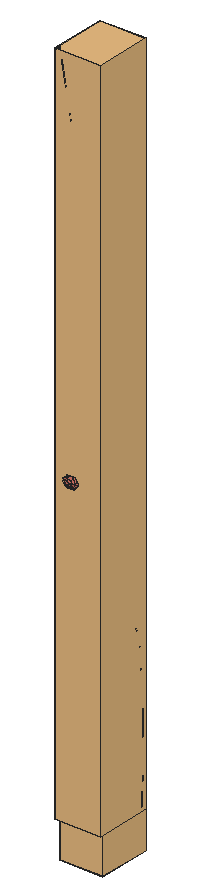
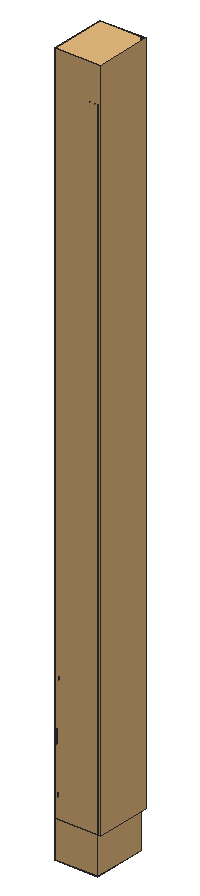
# SketchUp Ruby script. Lengths in inches.
U = 1.inch
M = Sketchup.active_model
def pt(a) = Geom::Point3d.new(a.map { |v| v * U })
def face(e, loops, mat)
  f = e.add_face(loops[0].map { |a| pt(a) })
  loops[1..].each { |l| e.add_face(l.map { |a| pt(a) }).erase! }
  f.material = f.back_material = mat if mat
  f
end
# faces: each face lists its corners as indices into pts; further lists are holes
def faces(e, pts, list, mat = nil) = list.each { |f| face(e, (f[0].is_a?(Array) ? f : [f]).map { |l| l.map { |i| pts[i] } }, mat) }
# xy, xz, yz: faces in a plane at the given z, y or x. An outline is a flat list of corners, or four numbers for a rectangle; further outlines are holes
def ring(l) = l.size == 4 ? [[l[0], l[1]], [l[2], l[1]], [l[2], l[3]], [l[0], l[3]]] : l.each_slice(2).to_a
def flat(e, list, mat, &to3) = list.each { |f| face(e, (f[0].is_a?(Array) ? f : [f]).map { |l| ring(l).map { |u, v| to3.(u, v) } }, mat) }
def xy(e, z, list, mat = nil) = flat(e, list, mat) { |x, y| [x, y, z] }
def xz(e, y, list, mat = nil) = flat(e, list, mat) { |x, z| [x, y, z] }
def yz(e, x, list, mat = nil) = flat(e, list, mat) { |y, z| [x, y, z] }
def lines(e, pts, list) = list.each { |a, b| e.add_line(pt(pts[a]), pt(pts[b])) }
# prism: a flat outline (further loops are holes) pulled along v
def prism(e, loops, v, mat = nil)
  f = face(e, loops, mat); d = Geom::Vector3d.new(v.map { |x| x * U })
  f.pushpull(f.normal.samedirection?(d) ? d.length : -d.length)
end
def box(e, o, s, mat = nil) = prism(e, [[o, [o[0] + s[0], o[1], o[2]], [o[0] + s[0], o[1] + s[1], o[2]], [o[0], o[1] + s[1], o[2]]]], [0, 0, s[2]], mat)
def at(x, y, z, deg = 0) = Geom::Transformation.translation(pt([x, y, z])) * Geom::Transformation.rotation(ORIGIN, Z_AXIS, deg.degrees)
def axes(o, x, y, z) = Geom::Transformation.new([*x, 0, *y, 0, *z, 0, *pt(o).to_a, 1])
def part(name) = M.definitions.add(name)
# library, detail: a bought-in or finely detailed component or shape, given as its bounding box
def library(name, o, s) = part(name).tap { |d| box(d.entities, o, s) }
def detail(e, o, s) = box(e.add_group.entities, o, s)
def put(e, d, t, mat = nil) = e.add_instance(d, t).tap { |i| i.material = mat if mat }
def group(e, t, mat = nil) = e.add_group.tap { |g| g.transformation = t; g.material = mat if mat }.entities
root = M.entities
M.materials.add("green").color = [174, 139, 102]
M.materials.add("vio").color = [206, 114, 100]
c1 = part("3DGeom~209_Defintion")
p = [[-82.63,99.78,-479.67],[16.24,-187.65,-448.99],[-197.0625,-62.73,-454.35],[148.38,0,-478.24],[-291.5,172.82,-352.58],[-2.625,262.29,-394.02],
  [-245.31,266.64,-303.125],[-291.5,172.82,-352.58],[-245.31,266.64,-303.125],[225.19,-262.29,-323.34],[339.63,-99.78,-348.66],[240.76,187.65,-379.34],
  [-120.25,-325.02,-299.44],[-315.27,-181.7,-324.83],[-120.25,-325.02,-299.44],[-357.57,78.99,-337.96],[-315.27,-181.7,-324.83],[-291.5,172.82,-352.58],
  [-357.57,78.99,-337.96],[106.99,-381.25,-193.82],[-120.25,-325.02,-299.44],[106.99,-381.25,-193.82],[21.51,381.25,-220.34],[-231.37,335.33,-202.85],
  [-2.625,262.29,-394.02],[-245.31,266.64,-303.125],[-231.37,335.33,-202.85],[21.51,381.25,-220.34],[-2.625,262.29,-394.02],[419.63,62.73,-263.01],
  [268.63,325.02,-178.79],[419.63,62.73,-263.01],[240.76,187.65,-379.34],[21.51,381.25,-220.34],[268.63,325.02,-178.79],[-291.5,172.82,-352.58],
  [-357.57,78.99,-337.96],[-422.26,199.55,-131.01],[-245.31,266.64,-303.125],[339.63,-99.78,-348.66],[373.81,-266.64,-111.04],[225.19,-262.29,-323.34],
  [339.63,-99.78,-348.66],[439.875,-172.82,-125.66],[373.81,-266.64,-111.04],[419.63,62.73,-263.01],[339.63,-99.78,-348.66],[-357.57,78.99,-337.96],
  [-315.27,-181.7,-324.83],[-425.81,10.31,-263.18],[-425.81,10.31,-263.18],[-315.27,-181.7,-324.83],[-224.52,-375.3,-69.66],[-405.57,-225.25,-125.83],
  [-315.27,-181.7,-324.83],[-120.25,-325.02,-299.44],[-315.27,-181.7,-324.83],[-405.57,-225.25,-125.83],[225.19,-262.29,-323.34],[305.5625,-335.33,-36.26],
  [106.99,-381.25,-193.82],[225.19,-262.29,-323.34],[373.81,-266.64,-111.04],[-231.37,335.33,-202.85],[16.69,-424.8,5.18],[-477.94,-14.83,-148.29],
  [419.63,62.73,-263.01],[486.07,-78.99,-76.21],[443.77,181.7,-89.33],[419.63,62.73,-263.01],[268.63,325.02,-178.79],[419.63,62.73,-263.01],
  [-16.69,424.8,-5.18],[268.63,325.02,-178.79],[-253.43,360.47,-78.63],[-231.37,335.33,-202.85],[-253.43,360.47,-78.63],[-253.43,360.47,-78.63],
  [253.43,-360.47,78.63],[224.52,375.3,69.66],[268.63,325.02,-178.79],[224.52,375.3,69.66],[268.63,325.02,-178.79],[-443.77,-181.7,89.33],
  [-500,10.31,-24.0625],[-486.07,78.99,76.21],[-439.875,172.82,125.66],[-373.81,266.64,111.04],[-305.5625,335.33,36.26],[-224.52,-375.3,-69.66],
  [-268.63,-325.02,178.79],[373.81,-266.64,-111.04],[422.26,-199.55,131.01],[305.5625,-335.33,-36.26],[373.81,-266.64,-111.04],[500,-10.31,24.0625],
  [405.57,225.25,125.83],[224.52,375.3,69.66],[-305.5625,335.33,36.26],[-253.43,360.47,-78.63],[-21.51,-381.25,220.34],[-21.51,-381.25,220.34],
  [-268.63,-325.02,178.79],[253.43,-360.47,78.63],[305.5625,-335.33,-36.26],[-419.63,-62.73,263.01],[-305.5625,335.33,36.26],[-106.99,381.25,193.82],
  [231.37,-335.33,202.85],[-21.51,-381.25,220.34],[477.94,14.83,148.29],[-373.81,266.64,111.04],[-305.5625,335.33,36.26],[120.25,325.02,299.44],
  [405.57,225.25,125.83],[-339.63,99.78,348.66],[231.37,-335.33,202.85],[253.43,-360.47,78.63],[-240.76,-187.65,379.34],[-240.76,-187.65,379.34],
  [-225.19,262.29,323.34],[-373.81,266.64,111.04],[-225.19,262.29,323.34],[-225.19,262.29,323.34],[315.27,181.7,324.83],[315.27,181.7,324.83],
  [405.57,225.25,125.83],[245.31,-266.64,303.125],[231.37,-335.33,202.85],[291.5,-172.82,352.58],[245.31,-266.64,303.125],[357.57,-78.99,337.96],
  [291.5,-172.82,352.58],[425.81,-10.31,263.18],[357.57,-78.99,337.96],[315.27,181.7,324.83],[-268.63,-325.02,178.79],[-21.51,-381.25,220.34],
  [2.625,-262.29,394.02],[-268.63,-325.02,178.79],[-240.76,-187.65,379.34],[-225.19,262.29,323.34],[120.25,325.02,299.44],[-106.99,381.25,193.82],
  [-21.51,-381.25,220.34],[245.31,-266.64,303.125],[-21.51,-381.25,220.34],[245.31,-266.64,303.125],[2.625,-262.29,394.02],[-419.63,-62.73,263.01],
  [-148.38,0,478.24],[-419.63,-62.73,263.01],[-339.63,99.78,348.66],[197.0625,62.74,454.35],[357.57,-78.99,337.96],[425.81,-10.31,263.18],
  [425.81,-10.31,263.18],[315.27,181.7,324.83],[-16.24,187.65,448.99],[315.27,181.7,324.83],[120.25,325.02,299.44],[-225.19,262.29,323.34],
  [120.25,325.02,299.44],[245.31,-266.64,303.125],[291.5,-172.82,352.58],[-339.63,99.78,348.66],[-225.19,262.29,323.34],[315.27,181.7,324.83],
  [82.63,-99.77,479.67],[-339.63,99.78,348.66]]
faces(c1.entities,p,[[0,1,2],[0,3,1],[4,0,2],[5,3,0],[6,0,7],[8,5,0],[3,9,1],[3,10,9],
  [11,10,3],[5,11,3],[2,12,13],[2,1,14],[15,2,16],[17,2,18],[1,19,20],[1,9,21],
  [22,11,5],[23,24,25],[26,27,28],[11,29,10],[30,31,32],[33,34,11],[35,36,37],[38,35,37],
  [39,40,41],[42,43,44],[45,43,46],[47,48,49],[36,50,37],[51,52,53],[54,55,52],[50,56,57],
  [58,59,60],[61,62,59],[63,38,37],[55,64,52],[55,60,64],[50,57,65],[50,65,37],[66,67,43],
  [68,67,69],[70,68,71],[72,73,27],[74,27,75],[76,72,27],[77,63,37],[60,78,64],[60,59,78],
  [79,68,80],[72,81,82],[65,57,83],[65,83,84],[65,84,37],[84,85,37],[85,86,37],[86,87,37],
  [88,77,37],[87,88,37],[57,89,90],[57,90,83],[91,43,92],[43,67,92],[93,94,92],[68,95,67],
  [96,95,68],[97,96,68],[98,72,99],[67,95,92],[52,64,100],[52,101,102],[103,104,92],[84,83,105],
  [84,105,85],[106,107,72],[107,81,72],[64,108,109],[64,78,108],[95,110,92],[96,110,95],[111,107,112],
  [113,114,81],[107,113,81],[85,105,115],[85,115,86],[116,117,92],[83,90,118],[83,119,105],[86,120,87],
  [121,122,107],[86,115,123],[124,110,96],[113,125,126],[127,128,92],[129,130,92],[131,132,92],[133,134,92],
  [110,133,92],[135,133,110],[136,137,138],[139,138,140],[141,142,143],[144,108,145],[146,147,148],[149,140,150],
  [151,150,152],[153,154,155],[153,156,157],[158,159,160],[161,158,162],[138,163,164],[165,158,166],[158,153,167],
  [168,164,154],[168,154,153],[169,150,158],[138,164,168],[140,138,168],[140,168,150],[150,153,158],[150,168,153]],"vio")
c2 = part("3DGeom~162_Defintion")
p = [[24.5,499.67,-28.18],[34.6875,499.96,-22.61],[27.51,499.8125,-29.5],[24.5,499.67,-28.18],[27.51,499.8125,-29.5],[25.94,499.74,-29.06],
  [27.51,499.8125,-29.5],[34.6875,499.96,-22.61],[30.68,499.93,-29.16],[27.51,499.8125,-29.5],[30.68,499.93,-29.16],[29.11,499.875,-29.54],
  [30.68,499.93,-29.16],[34.6875,499.96,-22.61],[33.33,499.99,-27.23],[30.68,499.93,-29.16],[33.33,499.99,-27.23],[32.11,499.97,-28.39],
  [22.58,499.54,-25.53],[34.6875,499.96,-22.61],[24.5,499.67,-28.18],[22.58,499.54,-25.53],[24.5,499.67,-28.18],[23.34,499.6,-26.96],
  [33.33,499.99,-27.23],[34.6875,499.96,-22.61],[34.66,499.99,-24.22],[33.33,499.99,-27.23],[34.66,499.99,-24.22],[34.21,500,-25.79],
  [22.24,499.47,-22.35],[34.6875,499.96,-22.61],[22.58,499.54,-25.53],[22.24,499.47,-22.35],[22.58,499.54,-25.53],[22.2,499.5,-23.96],
  [23.56,499.46,-19.35],[34.6875,499.96,-22.61],[22.24,499.47,-22.35],[26.22,499.53,-17.41],[34.6875,499.96,-22.61],[23.56,499.46,-19.35],
  [34.32,499.91,-21.05],[34.6875,499.96,-22.61],[26.22,499.53,-17.41],[23.56,499.46,-19.35],[22.24,499.47,-22.35],[22.6875,499.46,-20.79],
  [34.32,499.91,-21.05],[26.22,499.53,-17.41],[27.78,499.58,-17.04],[30.95,499.72,-17.52],[34.32,499.91,-21.05],[27.78,499.58,-17.04],
  [32.39,499.79,-18.39],[34.32,499.91,-21.05],[30.95,499.72,-17.52],[32.39,499.79,-18.39],[33.55,499.86,-19.61],[34.32,499.91,-21.05],
  [26.22,499.53,-17.41],[23.56,499.46,-19.35],[24.78,499.49,-18.1875],[30.95,499.72,-17.52],[27.78,499.58,-17.04],[29.39,499.65,-17.07],
  [-36.91,-499.89,26.6875],[-36.31,-499.93,26.63],[-35.71,-499.97,26.73],[-36.91,-499.89,26.6875],[-35.71,-499.97,26.73],[-34.01,-499.94,29.09],
  [-35.71,-499.97,26.73],[-35.15,-499.99,26.99],[-34.65,-500,27.39],[-35.71,-499.97,26.73],[-34.65,-500,27.39],[-34.01,-499.94,29.09],
  [-38,-499.78,27.26],[-37.49,-499.83,26.9],[-36.91,-499.89,26.6875],[-38,-499.78,27.26],[-36.91,-499.89,26.6875],[-34.01,-499.94,29.09],
  [-38.66,-499.67,28.32],[-38,-499.78,27.26],[-34.01,-499.94,29.09],[-38.66,-499.67,28.32],[-38.41,-499.72,27.75],[-38,-499.78,27.26],
  [-34.65,-500,27.39],[-34.29,-499.99,27.91],[-34.07,-499.97,28.49],[-34.65,-500,27.39],[-34.07,-499.97,28.49],[-34.01,-499.94,29.09],
  [-38.69,-499.59,29.52],[-38.66,-499.67,28.32],[-34.01,-499.94,29.09],[-38.69,-499.59,29.52],[-38.75,-499.625,28.91],[-38.66,-499.67,28.32],
  [-38.11,-499.57,30.62],[-38.69,-499.59,29.52],[-34.01,-499.94,29.09],[-37.06,-499.6,31.27],[-38.11,-499.57,30.62],[-34.01,-499.94,29.09],
  [-34.11,-499.9,29.69],[-37.06,-499.6,31.27],[-34.01,-499.94,29.09],[-38.11,-499.57,30.62],[-38.48,-499.57,30.1],[-38.69,-499.59,29.52],
  [-34.11,-499.9,29.69],[-36.46,-499.64,31.375],[-37.06,-499.6,31.27],[-35.28,-499.73,31.11],[-36.46,-499.64,31.375],[-34.11,-499.9,29.69],
  [-34.11,-499.9,29.69],[-34.76,-499.79,30.74],[-35.28,-499.73,31.11],[-34.11,-499.9,29.69],[-34.36,-499.85,30.25],[-34.76,-499.79,30.74],
  [-37.06,-499.6,31.27],[-37.62,-499.58,31.02],[-38.11,-499.57,30.62],[-35.28,-499.73,31.11],[-35.86,-499.68,31.32],[-36.46,-499.64,31.375]]
faces(c2.entities,p,[[0,1,2],[3,4,5],[6,7,8],[9,10,11],[12,13,14],[15,16,17],[18,19,20],[21,22,23],
  [24,25,26],[27,28,29],[30,31,32],[33,34,35],[36,37,38],[39,40,41],[42,43,44],[45,46,47],
  [48,49,50],[51,52,53],[54,55,56],[57,58,59],[60,61,62],[63,64,65],[66,67,68],[69,70,71],
  [72,73,74],[75,76,77],[78,79,80],[81,82,83],[84,85,86],[87,88,89],[90,91,92],[93,94,95],
  [96,97,98],[99,100,101],[102,103,104],[105,106,107],[108,109,110],[111,112,113],[114,115,116],[117,118,119],
  [120,121,122],[123,124,125],[126,127,128],[129,130,131]],"green")
c3 = library("3DGeom~76_Defintion",[-357.42,-500,-94.02],[714.84,1000,188.04])
c4 = part("3DGeom~77_Defintion")
p = [[339.625,495.99,-59.28],[344.32,486.75,-93.94],[336.28,491.02,-94.02],[339.625,495.99,-59.28],[336.28,491.02,-94.02],[329.77,495.38,-89.43],
  [339.625,495.99,-59.28],[351.73,483.72,-89.22],[344.32,486.75,-93.94],[339.625,495.99,-59.28],[329.77,495.38,-89.43],[326.53,498.67,-81.4],
  [339.625,495.99,-59.28],[356.52,482.74,-81.125],[351.73,483.72,-89.22],[339.625,495.99,-59.28],[326.53,498.67,-81.4],[327.42,500,-72.09],
  [339.625,495.99,-59.28],[357.42,484.07,-71.82],[356.52,482.74,-81.125],[339.625,495.99,-59.28],[327.42,500,-72.09],[332.22,499.02,-64],
  [339.625,495.99,-59.28],[354.18,487.36,-63.79],[357.42,484.07,-71.82],[339.625,495.99,-59.28],[347.66,491.72,-59.2],[354.18,487.36,-63.79],
  [-333.46,-489.29,27.51],[-350.37,-484.43,31.63],[-342.13,-486.03,27.33],[-323.61,-497.07,39.94],[-347.57,-495.14,60.61],[-333.46,-489.29,27.51],
  [-323.61,-497.07,39.94],[-333.46,-489.29,27.51],[-326.68,-493.33,32.125],[-333.46,-489.29,27.51],[-347.57,-495.14,60.61],[-350.37,-484.43,31.63],
  [-350.37,-484.43,31.63],[-347.57,-495.14,60.61],[-357.42,-487.36,48.18],[-350.37,-484.43,31.63],[-357.42,-487.36,48.18],[-355.96,-484.92,39.27],
  [-330.67,-500,56.48],[-347.57,-495.14,60.61],[-323.61,-497.07,39.94],[-330.67,-500,56.48],[-323.61,-497.07,39.94],[-325.07,-499.51,48.85],
  [-347.57,-495.14,60.61],[-354.35,-491.1,55.99],[-357.42,-487.36,48.18],[-347.57,-495.14,60.61],[-330.67,-500,56.48],[-338.9,-498.4,60.79]]
faces(c4.entities,p,[[0,1,2],[3,4,5],[6,7,8],[9,10,11],[12,13,14],[15,16,17],[18,19,20],[21,22,23],
  [24,25,26],[27,28,29],[30,31,32],[33,34,35],[36,37,38],[39,40,41],[42,43,44],[45,46,47],
  [48,49,50],[51,52,53],[54,55,56],[57,58,59]],"green")
c5 = library("3DGeom~161_Defintion",[-40.83,-526.88,-33.06],[81.66,1000,66.12])
c6 = library("3DGeom~158_Defintion",[-40.84,-526.87,-33.0625],[81.68,1000,66.125])
c7 = part("3DGeom~155_Defintion")
p = [[38.32,377.89,-31.94],[39.08,336.41,-30.625],[37.92,336.42,-31.72],[39.51,377.89,-30.8125],[36.28,473.1,-31.04],[39,423.46,-30.56],
  [37.77,423.45,-31.72],[36.57,299.05,-31.05],[35.37,265.71,-28.9],[34.28,265.75,-29.93],[37.7,299.02,-29.98],[37.54,473.12,-29.85],
  [30.51,238.44,-28.47],[26.13,217.53,-25.5625],[25.09,217.6875,-26.58],[31.58,238.34,-27.4375],[18.69,201.11,-24.24],[13.09,186.1875,-20.43],
  [12.09,186.36,-21.43],[19.71,200.92,-23.23],[17.34,-63.12,-14.97],[21.97,-83.66,-18.45],[21.09,-83.65,-19.17],[20.41,-107.24,-19.11],
  [17.68,-132.65,-15.82],[16.86,-132.61,-16.5],[21.25,-107.27,-18.41],[18.22,-63.09,-14.24],[5.95,170.98,-18.125],[1.85,152.3,-13.32],
  [0.82,152.32,-14.25],[6.97,170.87,-17.16],[11.42,-160.05,-12.18],[5.8,-189.86,-6.34],[5.02,-189.82,-6.98],[12.22,-160.09,-11.52],
  [-4.11,129.18,-8.57],[-8.33,104.16,-0.18],[-9.33,104.1,-1.06],[-3.09,129.2,-7.66],[0.27,-33.7,2.54],[10.55,-46.99,-6.22],
  [9.67,-47.04,-6.98],[1.16,-33.64,3.32],[-1.41,-222.19,-1.7],[-6.22,-257.42,3.45],[-6.96,-257.4,2.85],[-0.65,-222.22,-1.08],
  [-11.84,-295.59,6.88],[-16.11,-336.49,11.55],[-16.77,-336.48,11.01],[-11.14,-295.61,7.45],[-14.18,78.26,6.96],[-17,52.91,15.01],
  [-17.97,52.84,14.16],[-13.19,78.33,7.82],[-16.02,-7.84,18.13],[-7.97,-21.15,12.31],[-8.87,-21.22,11.51],[-15.1,-7.78,18.9375],
  [-21.76,-380.05,15.23],[-26.21,-426.32,20.02],[-26.8,-426.3,19.54],[-21.13,-380.0625,15.74],[-20.06,29.08,19.25],[-18.85,8.375,21.75],
  [-19.78,8.33,20.94],[-19.1,29.15,20.08],[-31.89,-475.25,23.94],[-36.52,-526.88,28.86],[-37.04,-526.87,28.4375],[-31.34,-475.26,24.4]]
faces(c7.entities,p,[[0,1,2],[0,3,1],[4,5,6],[7,8,9],[7,10,8],[4,11,5],[12,13,14],[12,15,13],
  [16,17,18],[16,19,17],[20,21,22],[23,24,25],[23,26,24],[20,27,21],[28,29,30],[28,31,29],
  [32,33,34],[32,35,33],[36,37,38],[36,39,37],[40,41,42],[40,43,41],[44,45,46],[44,47,45],
  [48,49,50],[48,51,49],[52,53,54],[52,55,53],[56,57,58],[56,59,57],[60,61,62],[60,63,61],
  [64,65,66],[64,67,65],[68,69,70],[68,71,69]],"green")
c8 = part("3DGeom~159_Defintion")
p = [[36.92,377.89,-32.7],[37.92,336.42,-31.72],[36.56,336.4375,-32.45],[38.32,377.89,-31.94],[34.8,473.07,-31.83],[37.77,423.44,-31.72],
  [36.34,423.43,-32.49],[35.25,299.08,-31.77],[34.28,265.75,-29.93],[32.99,265.81,-30.625],[36.57,299.05,-31.05],[36.28,473.1,-31.04],
  [39.51,377.89,-30.8125],[39.91,336.41,-29.26],[39.08,336.41,-30.625],[39.51,377.89,-30.8125],[40.37,377.89,-29.41],[37.53,473.12,-29.85],
  [39.87,423.46,-29.11],[39,423.45,-30.56],[37.7,299.02,-29.98],[36.15,265.7,-27.6],[35.37,265.71,-28.9],[37.7,299.02,-29.98],
  [38.51,299.02,-28.66],[37.53,473.12,-29.85],[38.43,473.12,-28.37],[29.25,238.59,-29.15],[25.09,217.6875,-26.58],[23.87,217.92,-27.27],
  [30.51,238.44,-28.47],[31.58,238.34,-27.4375],[26.875,217.45,-24.3],[26.13,217.52,-25.5625],[31.58,238.34,-27.4375],[32.35,238.29,-26.16],
  [17.52,201.39,-24.93],[12.09,186.36,-21.43],[10.92,186.63,-22.1],[18.69,201.11,-24.24],[19.71,200.92,-23.23],[13.83,186.13,-19.21],
  [13.09,186.1875,-20.43],[19.71,200.92,-23.23],[20.44,200.83,-21.98],[16.34,-63.24,-15.45],[21.09,-83.65,-19.17],[20.1,-83.67,-19.61],
  [19.4375,-107.2,-19.54],[16.86,-132.61,-16.5],[15.92,-132.54,-16.92],[20.41,-107.24,-19.11],[17.34,-63.12,-14.97],[4.77,171.17,-18.77],
  [0.82,152.32,-14.25],[-0.37,152.41,-14.87],[5.95,170.97,-18.125],[21.25,-107.27,-18.41],[18.3,-132.64,-14.94],[17.68,-132.65,-15.82],
  [21.25,-107.27,-18.41],[21.89,-107.28,-17.51],[18.22,-63.09,-14.24],[22.62,-83.68,-17.53],[21.97,-83.66,-18.45],[18.22,-63.09,-14.24],
  [18.89,-63.17,-13.31],[6.97,170.87,-17.16],[2.6,152.35,-12.15],[1.85,152.3,-13.32],[6.97,170.87,-17.16],[7.71,170.87,-15.96],
  [10.51,-159.96,-12.6],[5.02,-189.82,-6.98],[4.14,-189.74,-7.39],[11.42,-160.05,-12.18],[12.22,-160.09,-11.52],[6.39,-189.85,-5.52],
  [5.8,-189.86,-6.34],[12.22,-160.09,-11.52],[12.82,-160.08,-10.67],[-5.29,129.23,-9.17],[-9.33,104.1,-1.06],[-10.49,104.14,-1.64],
  [-4.11,129.17,-8.57],[-3.09,129.2,-7.66],[-7.59,104.3,0.93],[-8.33,104.16,-0.18],[-3.09,129.2,-7.66],[-2.34,129.3125,-6.53],
  [-0.69,-33.93,1.99],[9.67,-47.04,-6.98],[8.7,-47.23,-7.5],[0.27,-33.7,2.54],[1.16,-33.64,3.32],[11.25,-47.11,-5.29],
  [10.55,-46.99,-6.22],[1.16,-33.64,3.32],[1.875,-33.77,4.25],[-2.26,-222.12,-2.1],[-6.96,-257.4,2.85],[-7.79,-257.35,2.47],
  [-1.41,-222.19,-1.7],[-0.65,-222.22,-1.08],[-5.67,-257.41,4.22],[-6.22,-257.42,3.45],[-0.65,-222.22,-1.08],[-0.09,-222.21,-0.28],
  [-15.32,78.28,6.39],[-17.97,52.84,14.16],[-19.09,52.83,13.61],[-14.18,78.26,6.96],[-12.63,-295.55,6.52],[-16.77,-336.48,11.01],
  [-17.52,-336.4375,10.67],[-11.84,-295.59,6.88],[-11.14,-295.61,7.45],[-15.61,-336.49,12.25],[-16.11,-336.49,11.55],[-11.14,-295.61,7.45],
  [-10.62,-295.6,8.19],[-13.19,78.33,7.82],[-16.29,53.04,16.07],[-17,52.91,15.01],[-13.19,78.33,7.82],[-12.46,78.47,8.9],
  [-17.06,-8,17.6],[-8.87,-21.22,11.51],[-9.86,-21.4375,10.96],[-16.02,-7.84,18.13],[-15.1,-7.78,18.9375],[-7.26,-21.26,13.27],
  [-7.97,-21.15,12.31],[-15.1,-7.78,18.9375],[-14.41,-7.83,19.9375],[-22.47,-380.01,14.91],[-26.8,-426.3,19.54],[-27.47,-426.27,19.24],
  [-21.76,-380.05,15.23],[-21.13,-380.0625,15.74],[-25.76,-426.31,20.65],[-26.21,-426.32,20.02],[-21.13,-380.0625,15.74],[-20.66,-380.05,16.4],
  [-21.15,29.05,18.72],[-20.05,29.08,19.25],[-19.78,8.33,20.94],[-20.86,8.27,20.42],[-19.1,29.14,20.08],[-18.41,29.24,21.125],
  [-18.17,8.4,22.78],[-19.1,29.14,20.08],[-18.85,8.375,21.75],[-32.52,-475.22,23.66],[-37.04,-526.87,28.4375],[-37.63,-526.84,28.17],
  [-31.89,-475.24,23.94],[-31.33,-475.26,24.4],[-36.13,-526.875,29.41],[-36.52,-526.88,28.86],[-31.33,-475.26,24.4],[-30.92,-475.25,24.98]]
faces(c8.entities,p,[[0,1,2],[0,3,1],[4,5,6],[7,8,9],[7,10,8],[4,11,5],[12,13,14],[15,16,13],
  [17,18,19],[20,21,22],[23,24,21],[25,26,18],[27,28,29],[27,30,28],[31,32,33],[34,35,32],
  [36,37,38],[36,39,37],[40,41,42],[43,44,41],[45,46,47],[48,49,50],[48,51,49],[45,52,46],
  [53,54,55],[53,56,54],[57,58,59],[60,61,58],[62,63,64],[65,66,63],[67,68,69],[70,71,68],
  [72,73,74],[72,75,73],[76,77,78],[79,80,77],[81,82,83],[81,84,82],[85,86,87],[88,89,86],
  [90,91,92],[90,93,91],[94,95,96],[97,98,95],[99,100,101],[99,102,100],[103,104,105],[106,107,104],
  [108,109,110],[108,111,109],[112,113,114],[112,115,113],[116,117,118],[119,120,117],[121,122,123],[124,125,122],
  [126,127,128],[126,129,127],[130,131,132],[133,134,131],[135,136,137],[135,138,136],[139,140,141],[142,143,140],
  [144,145,146],[144,146,147],[148,149,150],[151,150,152],[153,154,155],[153,156,154],[157,158,159],[160,161,158]],"green")
c9 = part("3DGeom~240_Defintion")
p = [[-78.2,0,-500],[136.57,-186.02,-435.25],[-104.59,-107.4,-478.72],[182.28,0,-472.11],[-317.72,0,-393.91],[-104.59,107.4,-478.72],
  [11.71,-322.2,-334.53],[-176.68,-186.02,-420.57],[-176.68,186.02,-420.57],[136.57,186.02,-435.25],[341.14,-214.8,-275.16],[393.91,0,-317.72],
  [196.96,-372.05,-158.86],[196.96,-372.05,-158.86],[341.14,214.8,-275.16],[11.71,322.2,-334.54],[-158.86,-372.05,-196.96],[-275.16,-214.8,-341.14],
  [-275.16,214.8,-341.14],[-373.63,-186.02,-261.71],[-373.63,-186.02,-261.71],[-445.73,-107.4,-203.5625],[-317.72,0,-393.91],[-472.11,0,-182.28],
  [-317.72,0,-393.91],[-445.73,107.4,-203.5625],[-317.72,0,-393.91],[-373.63,186.02,-261.71],[-317.72,0,-393.91],[-373.63,186.02,-261.71],
  [-275.16,-214.8,-341.14],[-158.86,-372.05,-196.96],[-329.43,-322.2,-59.38],[-275.16,-214.8,-341.14],[-329.43,-322.2,-59.38],[-373.63,-186.02,-261.71],
  [-373.63,186.02,-261.71],[-158.86,372.04,-196.96],[-275.16,214.8,-341.14],[-158.86,372.04,-196.96],[11.71,-322.2,-334.53],[0,-429.6,0],
  [-158.86,-372.05,-196.96],[11.71,-322.2,-334.53],[196.96,-372.05,-158.86],[196.96,372.04,-158.86],[-158.86,372.04,-196.96],[196.96,372.04,-158.86],
  [11.71,322.2,-334.54],[393.91,0,-317.72],[454.3,-186.02,-41.34],[341.14,-214.8,-275.16],[393.91,0,-317.72],[500,0,-78.2],
  [341.14,214.8,-275.16],[393.91,0,-317.72],[341.14,-214.8,-275.16],[329.43,-322.2,59.38],[196.96,-372.05,-158.86],[341.14,-214.8,-275.16],
  [329.43,-322.2,59.38],[341.14,214.8,-275.16],[454.3,186.02,-41.34],[196.96,372.04,-158.86],[341.14,214.8,-275.16],[-329.43,-322.2,-59.38],
  [-454.3,-186.02,41.34],[-329.43,322.2,-59.38],[-373.63,186.02,-261.71],[-373.63,186.02,-261.71],[-329.43,322.2,-59.38],[-158.86,372.04,-196.96],
  [-500,0,78.2],[-454.3,186.02,41.34],[-329.43,322.2,-59.38],[-158.86,-372.05,-196.96],[-196.96,-372.04,158.86],[-158.86,-372.05,-196.96],
  [-196.96,-372.04,158.86],[-329.43,-322.2,-59.38],[0,429.6,0],[-158.86,372.04,-196.96],[-158.86,372.04,-196.96],[196.96,372.04,-158.86],
  [158.86,-372.04,196.96],[329.43,-322.2,59.38],[196.96,372.04,-158.86],[329.43,322.2,59.38],[329.43,322.2,59.38],[196.96,372.04,-158.86],
  [445.73,-107.4,203.5625],[472.11,0,182.28],[-196.96,-372.04,158.86],[-341.14,-214.8,275.16],[-196.96,372.05,158.86],[-329.43,322.2,-59.38],
  [-196.96,372.05,158.86],[373.63,-186.02,261.71],[329.43,-322.2,59.38],[373.63,-186.02,261.71],[445.73,107.4,203.5625],[-11.71,-322.2,334.54],
  [-196.96,-372.04,158.86],[-11.71,-322.2,334.54],[158.86,372.05,196.96],[329.43,322.2,59.38],[-393.91,0,317.72],[-341.14,214.8,275.16],
  [-196.96,372.05,158.86],[275.16,-214.8,341.14],[373.63,-186.02,261.71],[373.63,186.02,261.71],[373.63,186.02,261.71],[329.43,322.2,59.38],
  [-196.96,-372.04,158.86],[-136.57,-186.02,435.25],[-341.14,-214.8,275.16],[-196.96,-372.04,158.86],[-11.71,-322.2,334.54],[-341.14,214.8,275.16],
  [-11.71,322.2,334.53],[-196.96,372.05,158.86],[-11.71,322.2,334.53],[317.72,0,393.91],[317.72,0,393.91],[158.86,-372.04,196.96],
  [176.68,-186.02,420.57],[158.86,-372.04,196.96],[275.16,-214.8,341.14],[275.16,214.8,341.14],[373.63,186.02,261.71],[-11.71,322.2,334.53],
  [275.16,214.8,341.14],[158.86,372.05,196.96],[373.63,-186.02,261.71],[317.72,0,393.91],[317.72,0,393.91],[275.16,-214.8,341.14],
  [373.63,-186.02,261.71],[317.72,0,393.91],[373.63,186.02,261.71],[275.16,214.8,341.14],[-341.14,-214.8,275.16],[-182.28,0,472.11],
  [-393.91,0,317.72],[-341.14,-214.8,275.16],[-393.91,0,317.72],[-136.57,186.02,435.25],[-341.14,214.8,275.16],[-341.14,214.8,275.16],
  [-11.71,322.2,334.53],[-393.91,0,317.72],[104.59,-107.4,478.72],[176.68,186.02,420.57],[-11.71,322.2,334.53],[-11.71,322.2,334.53],
  [275.16,214.8,341.14],[275.16,-214.8,341.14],[275.16,214.8,341.14],[78.2,0,500],[104.59,107.4,478.72]]
faces(c9.entities,p,[[0,1,2],[0,3,1],[0,2,4],[5,0,4],[5,3,0],[2,6,7],[2,1,6],[2,7,4],
  [8,5,4],[5,9,3],[8,9,5],[3,10,1],[3,11,10],[9,11,3],[1,12,6],[1,10,13],
  [9,14,11],[8,15,9],[15,14,9],[7,16,17],[7,6,16],[7,17,4],[18,8,4],[18,15,8],
  [17,19,4],[20,21,22],[21,23,24],[23,25,26],[25,27,28],[29,18,4],[30,31,32],[33,34,35],
  [36,37,38],[18,39,15],[40,41,42],[43,44,41],[15,45,14],[46,47,48],[49,50,51],[52,53,50],
  [54,53,55],[56,57,58],[59,50,60],[61,62,53],[63,62,64],[20,65,66],[20,66,21],[25,67,68],
  [69,70,71],[21,66,72],[21,72,23],[23,73,25],[25,73,74],[75,41,76],[77,78,79],[70,80,81],
  [82,80,83],[23,72,73],[44,84,41],[44,85,84],[86,87,62],[80,88,89],[53,90,50],[53,91,90],
  [62,91,53],[65,92,93],[65,93,66],[73,94,95],[70,96,80],[50,97,98],[50,90,99],[62,100,91],
  [87,100,62],[41,101,102],[41,84,103],[80,104,105],[96,104,80],[66,93,106],[66,106,72],[72,107,73],
  [73,107,108],[85,109,84],[85,110,109],[87,111,100],[104,112,113],[72,106,107],[114,115,116],[117,118,115],
  [119,120,121],[96,122,104],[90,91,123],[91,100,124],[125,126,118],[127,128,126],[104,129,130],[131,132,133],
  [134,90,135],[100,111,136],[137,138,139],[140,141,139],[142,143,144],[145,115,143],[146,147,148],[149,147,150],
  [151,143,147],[118,152,115],[118,126,152],[147,153,154],[155,153,156],[126,157,139],[158,153,139],[152,126,139],
  [159,152,139],[160,159,139],[153,160,139],[147,160,153],[115,159,143],[115,152,159],[143,160,147],[143,159,160]],"vio")
c10 = library("3DGeom~160_Defintion",[-35.87,-474.24,-32.99],[76.62,1000,62.39])
c11 = library("3DGeom~156_Defintion",[-35.87,-474.23,-32.99],[76.62,1000,62.39])
c12 = part("3DGeom~154_Defintion")
p = [[37.69,422.55,-31.65],[39.43,377.09,-30.75],[38.24,377.08,-31.875],[37.84,335.71,-31.66],[37.62,298.39,-29.92],[36.5,298.41,-30.99],
  [39,335.7,-30.56],[38.91,422.56,-30.49],[33.77,525.73,-29.85],[37.46,472.11,-29.79],[36.2,472.09,-30.97],[34.2,265.19,-29.87],
  [31.51,237.83,-27.38],[30.44,237.9375,-28.41],[35.3,265.15,-28.83],[35.05,525.75,-28.63],[25.03,217.23,-26.53],[19.66,200.49,-23.18],
  [18.65,200.68,-24.19],[26.07,217.0625,-25.51],[12.06,185.97,-21.38],[6.95,170.51,-17.12],[5.93,170.61,-18.08],[13.07,185.79,-20.39],
  [21.05,-83.47,-19.125],[21.21,-107.04,-18.37],[20.36,-107.02,-19.07],[21.92,-83.48,-18.41],[16.82,-132.33,-16.46],[12.19,-159.75,-11.49],
  [11.4,-159.71,-12.15],[17.65,-132.37,-15.78],[9.65,-46.9375,-6.96],[18.18,-62.96,-14.21],[17.3,-62.98,-14.9375],[10.53,-46.89,-6.21],
  [0.82,152,-14.22],[-3.09,128.93,-7.65],[-4.1,128.9,-8.55],[1.84,151.98,-13.29],[5.01,-189.42,-6.97],[-0.65,-221.75,-1.08],
  [-1.4,-221.72,-1.7],[5.79,-189.46,-6.32],[-9.3125,103.88,-1.06],[-13.16,78.16,7.8],[-14.15,78.09,6.94],[-8.3125,103.94,-0.18],
  [-8.85,-21.17,11.49],[1.16,-33.57,3.31],[0.27,-33.63,2.53],[-6.94,-256.85,2.84],[-11.11,-294.98,7.4375],[-11.81,-294.96,6.87],
  [-6.21,-256.87,3.44],[-7.96,-21.11,12.28],[-16.73,-335.76,10.98],[-21.09,-379.25,15.71],[-21.71,-379.24,15.19],[-16.07,-335.78,11.53],
  [-17.94,52.72,14.13],[-19.0625,29.08,20.03],[-20.01,29.02,19.21],[-16.97,52.79,14.98],[-19.74,8.3125,20.9],[-15.07,-7.76,18.9],
  [-15.98,-7.82,18.1],[-18.8125,8.36,21.71],[-26.74,-425.4,19.5],[-31.27,-474.25,24.35],[-31.82,-474.23,23.89],[-26.15,-425.41,19.98]]
faces(c12.entities,p,[[0,1,2],[3,4,5],[3,6,4],[0,7,1],[8,9,10],[11,12,13],[11,14,12],[8,15,9],
  [16,17,18],[16,19,17],[20,21,22],[20,23,21],[24,25,26],[24,27,25],[28,29,30],[28,31,29],
  [32,33,34],[32,35,33],[36,37,38],[36,39,37],[40,41,42],[40,43,41],[44,45,46],[44,47,45],
  [48,49,50],[51,52,53],[51,54,52],[48,55,49],[56,57,58],[56,59,57],[60,61,62],[60,63,61],
  [64,65,66],[64,67,65],[68,69,70],[68,71,69]],"green")
g1 = group(root,at(15.3125,134.49,26.21))
put(g1,c1,axes([-1.13,-0.59,9.41],[0,0.00039,0],[0,0,-0.00039],[-0.00039,0,0]),"vio")
put(root,c2,axes([14.3,134.2,35.93],[0,0.01161,0],[0,0,-0.01161],[-0.01161,0,0]),"green")
g2 = group(root,at(15.3125,134.49,26.21))
put(g2,c3,axes([-1.1,-0.3,8.98],[0,0.00081,0],[0,0,-0.00081],[-0.00081,0,0]),"green")
put(g2,c4,axes([-1.1,-0.3,8.98],[0,0.00081,0],[0,0,-0.00081],[-0.00081,0,0]),"green")
put(root,c5,axes([14.3,134.2,35.93],[0,0.01102,0],[0,0,-0.01102],[-0.01102,0,0]),"green")
put(root,c6,axes([14.3,134.2,35.93],[0,0.01102,0],[0,0,-0.01102],[-0.01102,0,0]),"green")
put(root,c7,axes([14.3,134.2,35.93],[0,0.01102,0],[0,0,-0.01102],[-0.01102,0,0]),"green")
put(root,c8,axes([14.3,134.2,35.93],[0,0.01102,0],[0,0,-0.01102],[-0.01102,0,0]),"green")
g3 = group(root,at(15.3125,134.49,26.21))
put(g3,c9,axes([-0.96,-0.26,8.41],[0,0.00039,0],[0,0,-0.00039],[-0.00039,0,0]),"vio")
put(root,c10,axes([14.3,134.2,35.93],[0,0.01104,0],[0,0,-0.01104],[-0.01104,0,0]),"green")
put(root,c11,axes([14.3,134.2,35.93],[0,0.01104,0],[0,0,-0.01104],[-0.01104,0,0]),"green")
put(root,c12,axes([14.3,134.2,35.93],[0,0.01104,0],[0,0,-0.01104],[-0.01104,0,0]),"green")
